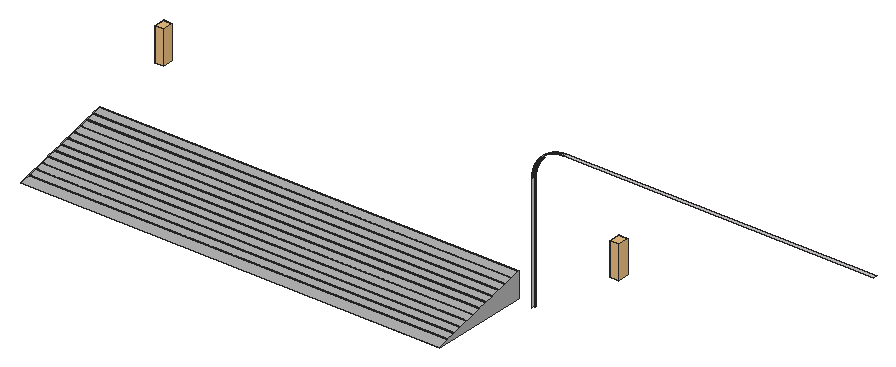
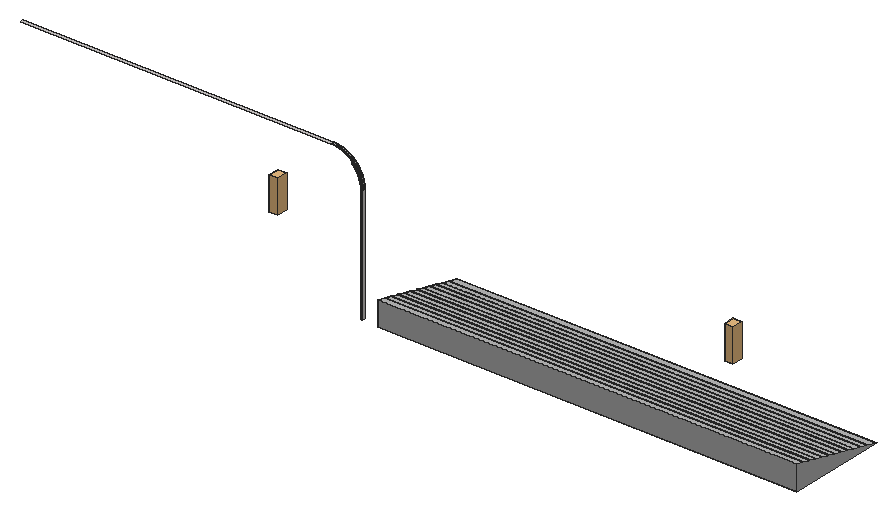
# SketchUp Ruby script. Lengths in inches.
U = 1.inch
M = Sketchup.active_model
def pt(a) = Geom::Point3d.new(a.map { |v| v * U })
def face(e, loops, mat)
  f = e.add_face(loops[0].map { |a| pt(a) })
  loops[1..].each { |l| e.add_face(l.map { |a| pt(a) }).erase! }
  f.material = f.back_material = mat if mat
  f
end
# faces: each face lists its corners as indices into pts; further lists are holes
def faces(e, pts, list, mat = nil) = list.each { |f| face(e, (f[0].is_a?(Array) ? f : [f]).map { |l| l.map { |i| pts[i] } }, mat) }
# xy, xz, yz: faces in a plane at the given z, y or x. An outline is a flat list of corners, or four numbers for a rectangle; further outlines are holes
def ring(l) = l.size == 4 ? [[l[0], l[1]], [l[2], l[1]], [l[2], l[3]], [l[0], l[3]]] : l.each_slice(2).to_a
def flat(e, list, mat, &to3) = list.each { |f| face(e, (f[0].is_a?(Array) ? f : [f]).map { |l| ring(l).map { |u, v| to3.(u, v) } }, mat) }
def xy(e, z, list, mat = nil) = flat(e, list, mat) { |x, y| [x, y, z] }
def xz(e, y, list, mat = nil) = flat(e, list, mat) { |x, z| [x, y, z] }
def yz(e, x, list, mat = nil) = flat(e, list, mat) { |y, z| [x, y, z] }
def lines(e, pts, list) = list.each { |a, b| e.add_line(pt(pts[a]), pt(pts[b])) }
# prism: a flat outline (further loops are holes) pulled along v
def prism(e, loops, v, mat = nil)
  f = face(e, loops, mat); d = Geom::Vector3d.new(v.map { |x| x * U })
  f.pushpull(f.normal.samedirection?(d) ? d.length : -d.length)
end
def box(e, o, s, mat = nil) = prism(e, [[o, [o[0] + s[0], o[1], o[2]], [o[0] + s[0], o[1] + s[1], o[2]], [o[0], o[1] + s[1], o[2]]]], [0, 0, s[2]], mat)
def at(x, y, z, deg = 0) = Geom::Transformation.translation(pt([x, y, z])) * Geom::Transformation.rotation(ORIGIN, Z_AXIS, deg.degrees)
def axes(o, x, y, z) = Geom::Transformation.new([*x, 0, *y, 0, *z, 0, *pt(o).to_a, 1])
def part(name) = M.definitions.add(name)
# library, detail: a bought-in or finely detailed component or shape, given as its bounding box
def library(name, o, s) = part(name).tap { |d| box(d.entities, o, s) }
def detail(e, o, s) = box(e.add_group.entities, o, s)
def put(e, d, t, mat = nil) = e.add_instance(d, t).tap { |i| i.material = mat if mat }
def group(e, t, mat = nil) = e.add_group.tap { |g| g.transformation = t; g.material = mat if mat }.entities
root = M.entities
M.materials.add("[Stone Vein Gray]").color = [206, 202, 201]
M.materials.add("[Terrazzo Tile Light]").color = [178, 178, 178]
c1 = library("WALL LIGHT 69",[4.19,4.05,-8.78],[4.61,5.7,17.13])
xy(root,0.35,[[172.85,83.25,173.15,83.5]])
xy(root,53.48,[[183.25,82.5,183.4,83.5]],"[Stone Vein Gray]")
xy(root,53.5,[[183.7,82.5,183.85,83.5],[183.85,82.5,184,83.5],[184,82.5,297,83.5]],"[Stone Vein Gray]")
xz(root,83.25,[[172.85,0,173.15,0.35]])
yz(root,172.5,[[82.5,0,83.5,42],[82.5,42,83.5,42.15],[82.5,42.15,83.5,42.3]],"[Stone Vein Gray]")
yz(root,172.52,[[82.5,42.6,83.5,42.75]],"[Stone Vein Gray]")
yz(root,172.85,[[83.25,0,83.5,0.35],[83.25,0.35,83.5,42],[83.25,42,83.5,42.15],[83.25,42.15,83.5,42.29]])
yz(root,173.15,[[83.25,0,83.5,0.35],[83.25,0.35,83.5,42],[83.25,42,83.5,42.14],[83.25,42.14,83.5,42.28]])
yz(root,173.16,[[83.25,42.43,83.5,42.57]])
p = [[172.51,83.5,42.45],[172.5,83.5,42.3],[172.5,82.5,42.3],[172.51,82.5,42.45],[172.85,83.5,42.29],[172.86,83.5,42.4375],
  [172.86,83.25,42.4375],[172.85,83.25,42.29],[173.16,83.5,42.43],[173.15,83.5,42.28],[173.15,83.25,42.28],[173.16,83.25,42.43],
  [172.87,83.5,42.58],[172.87,83.25,42.58],[172.52,83.5,42.6],[172.52,82.5,42.6],[172.875,83.5,42.73],[172.875,83.25,42.73],
  [173.17,83.5,42.71],[173.16,83.5,42.57],[173.16,83.25,42.57],[173.17,83.25,42.71],[172.88,83.5,42.875],[172.88,83.25,42.875],
  [173.18,83.5,42.85],[173.18,83.25,42.85],[172.54,83.5,42.9],[172.52,83.5,42.75],[172.52,82.5,42.75],[172.54,82.5,42.9],
  [172.55,83.5,43.05],[172.55,82.5,43.05],[172.9,83.5,43.02],[172.9,83.25,43.02],[173.2,83.5,42.99],[173.2,83.25,42.99],
  [172.91,83.5,43.17],[172.91,83.25,43.17],[173.21,83.5,43.13],[173.21,83.25,43.13],[172.5625,83.5,43.2],[172.5625,82.5,43.2],
  [173.23,83.5,43.28],[173.23,83.25,43.28],[172.58,83.5,43.35],[172.58,82.5,43.35],[172.93,83.5,43.3125],[172.93,83.25,43.3125],
  [172.95,83.5,43.46],[172.95,83.25,43.46],[173.24,83.5,43.42],[173.24,83.25,43.42],[172.6,83.5,43.5],[172.6,82.5,43.5],
  [173.26,83.5,43.56],[173.26,83.25,43.56],[172.62,83.5,43.65],[172.62,82.5,43.65],[172.97,83.5,43.6],[172.97,83.25,43.6],
  [172.99,83.5,43.74],[172.99,83.25,43.74],[173.28,83.5,43.7],[173.28,83.25,43.7],[172.64,83.5,43.8],[172.64,82.5,43.8],
  [173.01,83.5,43.89],[173.01,83.25,43.89],[173.31,83.5,43.84],[173.31,83.25,43.84],[172.67,83.5,43.95],[172.67,82.5,43.95],
  [173.33,83.5,43.98],[173.33,83.25,43.98],[172.69,83.5,44.1],[172.69,82.5,44.1],[173.04,83.5,44.03],[173.04,83.25,44.03],
  [173.0625,83.5,44.18],[173.0625,83.25,44.18],[173.36,83.5,44.12],[173.36,83.25,44.12],[172.72,83.5,44.24],[172.72,82.5,44.24],
  [173.39,83.5,44.26],[173.39,83.25,44.26],[172.75,83.5,44.39],[172.75,82.5,44.39],[173.09,83.5,44.32],[173.09,83.25,44.32],
  [173.125,83.5,44.46],[173.125,83.25,44.46],[173.42,83.5,44.39],[173.42,83.25,44.39],[172.78,83.5,44.54],[172.78,82.5,44.54],
  [173.45,83.5,44.53],[173.45,83.25,44.53],[172.82,83.5,44.68],[172.82,82.5,44.68],[173.16,83.5,44.6],[173.16,83.25,44.6],
  [173.48,83.5,44.67],[173.48,83.25,44.67],[173.19,83.5,44.74],[173.19,83.25,44.74],[172.85,83.5,44.83],[172.85,82.5,44.83],
  [173.23,83.5,44.89],[173.23,83.25,44.89],[173.52,83.5,44.81],[173.52,83.25,44.81],[172.89,83.5,44.98],[172.89,82.5,44.98],
  [173.56,83.5,44.95],[173.56,83.25,44.95],[173.27,83.5,45.03],[173.27,83.25,45.03],[173.6,83.5,45.08],[173.6,83.25,45.08],
  [172.93,83.5,45.12],[172.93,82.5,45.12],[173.31,83.5,45.17],[173.31,83.25,45.17],[172.97,83.5,45.27],[172.97,82.5,45.27],
  [173.64,83.5,45.22],[173.64,83.25,45.22],[173.35,83.5,45.31],[173.35,83.25,45.31],[173.68,83.5,45.35],[173.68,83.25,45.35],
  [173.02,83.5,45.41],[173.02,82.5,45.41],[173.4,83.5,45.45],[173.4,83.25,45.45],[173.0625,83.5,45.55],[173.0625,82.5,45.55],
  [173.44,83.5,45.58],[173.44,83.25,45.58],[173.73,83.5,45.49],[173.73,83.25,45.49],[173.77,83.5,45.62],[173.77,83.25,45.62],
  [173.11,83.5,45.7],[173.11,82.5,45.7],[173.49,83.5,45.72],[173.49,83.25,45.72],[173.82,83.5,45.76],[173.82,83.25,45.76],
  [173.16,83.5,45.84],[173.16,82.5,45.84],[173.54,83.5,45.86],[173.54,83.25,45.86],[173.21,83.5,45.98],[173.21,82.5,45.98],
  [173.87,83.5,45.89],[173.87,83.25,45.89],[173.59,83.5,46],[173.59,83.25,46],[173.92,83.5,46.02],[173.92,83.25,46.02],
  [173.26,83.5,46.12],[173.26,82.5,46.12],[173.64,83.5,46.13],[173.64,83.25,46.13],[173.98,83.5,46.15],[173.98,83.25,46.15],
  [173.32,83.5,46.26],[173.32,82.5,46.26],[173.7,83.5,46.27],[173.7,83.25,46.27],[174.03,83.5,46.28],[174.03,83.25,46.28],
  [173.375,83.5,46.4],[173.375,82.5,46.4],[173.76,83.5,46.4],[173.76,83.25,46.4],[174.09,83.5,46.41],[174.09,83.25,46.41],
  [173.43,83.5,46.54],[173.43,82.5,46.54],[173.8125,83.5,46.54],[173.8125,83.25,46.54],[174.15,83.5,46.54],[174.15,83.25,46.54],
  [173.49,83.5,46.68],[173.49,82.5,46.68],[173.875,83.5,46.67],[173.875,83.25,46.67],[174.21,83.5,46.67],[174.21,83.25,46.67],
  [173.56,83.5,46.81],[173.56,82.5,46.81],[173.9375,83.5,46.8],[173.9375,83.25,46.8],[174.27,83.5,46.8],[174.27,83.25,46.8],
  [173.62,83.5,46.95],[173.62,82.5,46.95],[174,83.5,46.93],[174,83.25,46.93],[174.33,83.5,46.93],[174.33,83.25,46.93],
  [174.07,83.5,47.0625],[174.07,83.25,47.0625],[174.4,83.5,47.05],[174.4,83.25,47.05],[173.6875,83.5,47.09],[173.6875,82.5,47.09],
  [173.75,83.5,47.22],[173.75,82.5,47.22],[174.13,83.5,47.19],[174.13,83.25,47.19],[174.46,83.5,47.18],[174.46,83.25,47.18],
  [173.82,83.5,47.35],[173.82,82.5,47.35],[174.2,83.5,47.32],[174.2,83.25,47.32],[174.53,83.5,47.3],[174.53,83.25,47.3],
  [174.27,83.5,47.45],[174.27,83.25,47.45],[174.6,83.5,47.42],[174.6,83.25,47.42],[173.89,83.5,47.49],[173.89,82.5,47.49],
  [174.34,83.5,47.57],[174.34,83.25,47.57],[174.68,83.5,47.55],[174.68,83.25,47.55],[173.97,83.5,47.62],[173.97,82.5,47.62],
  [174.75,83.5,47.67],[174.75,83.25,47.67],[174.04,83.5,47.75],[174.04,82.5,47.75],[174.42,83.5,47.7],[174.42,83.25,47.7],
  [174.49,83.5,47.83],[174.49,83.25,47.83],[174.82,83.5,47.79],[174.82,83.25,47.79],[174.12,83.5,47.88],[174.12,82.5,47.88],
  [174.57,83.5,47.95],[174.57,83.25,47.95],[174.9,83.5,47.91],[174.9,83.25,47.91],[174.19,83.5,48.01],[174.19,82.5,48.01],
  [174.65,83.5,48.07],[174.65,83.25,48.07],[174.98,83.5,48.03],[174.98,83.25,48.03],[174.27,83.5,48.14],[174.27,82.5,48.14],
  [175.06,83.5,48.15],[175.06,83.25,48.15],[174.36,83.5,48.26],[174.36,82.5,48.26],[174.73,83.5,48.19],[174.73,83.25,48.19],
  [175.14,83.5,48.26],[175.14,83.25,48.26],[174.8125,83.5,48.32],[174.8125,83.25,48.32],[174.4375,83.5,48.39],[174.4375,82.5,48.39],
  [174.89,83.5,48.44],[174.89,83.25,48.44],[175.22,83.5,48.38],[175.22,83.25,48.38],[174.52,83.5,48.51],[174.52,82.5,48.51],
  [174.98,83.5,48.55],[174.98,83.25,48.55],[175.31,83.5,48.49],[175.31,83.25,48.49],[174.61,83.5,48.64],[174.61,82.5,48.64],
  [175.39,83.5,48.61],[175.39,83.25,48.61],[174.7,83.5,48.76],[174.7,82.5,48.76],[175.07,83.5,48.67],[175.07,83.25,48.67],
  [175.48,83.5,48.72],[175.48,83.25,48.72],[175.15,83.5,48.79],[175.15,83.25,48.79],[175.57,83.5,48.83],[175.57,83.25,48.83],
  [174.79,83.5,48.88],[174.79,82.5,48.88],[175.24,83.5,48.9],[175.24,83.25,48.9],[175.66,83.5,48.9375],[175.66,83.25,48.9375],
  [174.875,83.5,49],[174.875,82.5,49],[175.33,83.5,49.02],[175.33,83.25,49.02],[175.75,83.5,49.05],[175.75,83.25,49.05],
  [174.97,83.5,49.12],[174.97,82.5,49.12],[175.43,83.5,49.13],[175.43,83.25,49.13],[175.84,83.5,49.15],[175.84,83.25,49.15],
  [175.0625,83.5,49.24],[175.0625,82.5,49.24],[175.52,83.5,49.24],[175.52,83.25,49.24],[175.16,83.5,49.35],[175.16,82.5,49.35],
  [175.62,83.5,49.35],[175.62,83.25,49.35],[175.9375,83.5,49.26],[175.9375,83.25,49.26],[176.03,83.5,49.36],[176.03,83.25,49.36],
  [175.26,83.5,49.47],[175.26,82.5,49.47],[175.71,83.5,49.46],[175.71,83.25,49.46],[176.13,83.5,49.47],[176.13,83.25,49.47],
  [175.35,83.5,49.58],[175.35,82.5,49.58],[175.8125,83.5,49.57],[175.8125,83.25,49.57],[176.23,83.5,49.57],[176.23,83.25,49.57],
  [175.45,83.5,49.7],[175.45,82.5,49.7],[175.91,83.5,49.68],[175.91,83.25,49.68],[176.33,83.5,49.67],[176.33,83.25,49.67],
  [175.56,83.5,49.81],[175.56,82.5,49.81],[176.01,83.5,49.78],[176.01,83.25,49.78],[176.43,83.5,49.77],[176.43,83.25,49.77],
  [175.66,83.5,49.92],[175.66,82.5,49.92],[176.53,83.5,49.87],[176.53,83.25,49.87],[175.76,83.5,50.02],[175.76,82.5,50.02],
  [175.87,83.5,50.13],[175.87,82.5,50.13],[175.98,83.5,50.24],[175.98,82.5,50.24],[176.08,83.5,50.34],[176.08,82.5,50.34],
  [176.19,83.5,50.44],[176.19,82.5,50.44],[176.3,83.5,50.55],[176.3,82.5,50.55],[176.42,83.5,50.65],[176.42,82.5,50.65],
  [176.53,83.5,50.74],[176.53,82.5,50.74],[176.65,83.5,50.84],[176.65,82.5,50.84],[176.76,83.5,50.9375],[176.76,82.5,50.9375],
  [176.88,83.5,51.03],[176.88,82.5,51.03],[177,83.5,51.125],[177,82.5,51.125],[177.12,83.5,51.21],[177.12,82.5,51.21],
  [177.24,83.5,51.3],[177.24,82.5,51.3],[177.36,83.5,51.39],[177.36,82.5,51.39],[177.49,83.5,51.48],[177.49,82.5,51.48],
  [177.61,83.5,51.5625],[177.61,82.5,51.5625],[177.74,83.5,51.64],[177.74,82.5,51.64],[177.86,83.5,51.73],[177.86,82.5,51.73],
  [177.99,83.5,51.81],[177.99,82.5,51.81],[178.12,83.5,51.88],[178.12,82.5,51.88],[178.25,83.5,51.96],[178.25,82.5,51.96],
  [178.38,83.5,52.03],[178.38,82.5,52.03],[178.51,83.5,52.11],[178.51,82.5,52.11],[178.65,83.5,52.18],[178.65,82.5,52.18],
  [178.78,83.5,52.25],[178.78,82.5,52.25],[178.91,83.5,52.3125],[178.91,82.5,52.3125],[179.05,83.5,52.38],[179.05,82.5,52.38],
  [179.19,83.5,52.44],[179.19,82.5,52.44],[179.32,83.5,52.51],[179.32,82.5,52.51],[179.46,83.5,52.57],[179.46,82.5,52.57],
  [179.6,83.5,52.625],[179.6,82.5,52.625],[179.74,83.5,52.68],[179.74,82.5,52.68],[179.88,83.5,52.74],[179.88,82.5,52.74],
  [180.02,83.5,52.79],[180.02,82.5,52.79],[180.16,83.5,52.84],[180.16,82.5,52.84],[180.3,83.5,52.89],[180.3,82.5,52.89],
  [180.45,83.5,52.9375],[180.45,82.5,52.9375],[180.59,83.5,52.98],[180.59,82.5,52.98],[180.73,83.5,53.03],[180.73,82.5,53.03],
  [180.88,83.5,53.07],[180.88,82.5,53.07],[181.02,83.5,53.11],[181.02,82.5,53.11],[181.17,83.5,53.15],[181.17,82.5,53.15],
  [181.32,83.5,53.18],[181.32,82.5,53.18],[181.46,83.5,53.22],[181.46,82.5,53.22],[181.61,83.5,53.25],[181.61,82.5,53.25],
  [181.76,83.5,53.28],[181.76,82.5,53.28],[181.9,83.5,53.31],[181.9,82.5,53.31],[182.05,83.5,53.33],[182.05,82.5,53.33],
  [182.2,83.5,53.36],[182.2,82.5,53.36],[182.35,83.5,53.38],[182.35,82.5,53.38],[182.5,83.5,53.4],[182.5,82.5,53.4],
  [182.65,83.5,53.42],[182.65,82.5,53.42],[182.8,83.5,53.4375],[182.8,82.5,53.4375],[182.95,83.5,53.45],[182.95,82.5,53.45],
  [183.1,83.5,53.46],[183.1,82.5,53.46],[183.25,83.5,53.48],[183.25,82.5,53.48],[183.55,83.5,53.49],[183.4,83.5,53.48],
  [183.4,82.5,53.48],[183.55,82.5,53.49],[183.7,83.5,53.5],[183.7,82.5,53.5]]
faces(root,p,[[0,1,2,3],[14,0,3,15],[26,27,28,29],[30,26,29,31],[40,30,31,41],[44,40,41,45],[52,44,45,53],[56,52,53,57],
  [64,56,57,65],[70,64,65,71],[74,70,71,75],[82,74,75,83],[86,82,83,87],[94,86,87,95],[98,94,95,99],[106,98,99,107],
  [112,106,107,113],[120,112,113,121],[124,120,121,125],[132,124,125,133],[136,132,133,137],[144,136,137,145],[150,144,145,151],[154,150,151,155],
  [162,154,155,163],[168,162,163,169],[174,168,169,175],[180,174,175,181],[186,180,181,187],[192,186,187,193],[198,192,193,199],[208,198,199,209],
  [210,208,209,211],[216,210,211,217],[226,216,217,227],[232,226,227,233],[236,232,233,237],[244,236,237,245],[250,244,245,251],[256,250,251,257],
  [260,256,257,261],[268,260,261,269],[274,268,269,275],[280,274,275,281],[284,280,281,285],[294,284,285,295],[300,294,295,301],[306,300,301,307],
  [312,306,307,313],[316,312,313,317],[324,316,317,325],[330,324,325,331],[336,330,331,337],[342,336,337,343],[348,342,343,349],[352,348,349,353],
  [354,352,353,355],[356,354,355,357],[358,356,357,359],[360,358,359,361],[362,360,361,363],[364,362,363,365],[366,364,365,367],[368,366,367,369],
  [370,368,369,371],[372,370,371,373],[374,372,373,375],[376,374,375,377],[378,376,377,379],[380,378,379,381],[382,380,381,383],[384,382,383,385],
  [386,384,385,387],[388,386,387,389],[390,388,389,391],[392,390,391,393],[394,392,393,395],[396,394,395,397],[398,396,397,399],[400,398,399,401],
  [402,400,401,403],[404,402,403,405],[406,404,405,407],[408,406,407,409],[410,408,409,411],[412,410,411,413],[414,412,413,415],[416,414,415,417],
  [418,416,417,419],[420,418,419,421],[422,420,421,423],[424,422,423,425],[426,424,425,427],[428,426,427,429],[430,428,429,431],[432,430,431,433],
  [434,432,433,435],[436,434,435,437],[438,436,437,439],[440,438,439,441],[442,440,441,443],[444,442,443,445],[446,444,445,447],[448,446,447,449],
  [450,448,449,451],[452,450,451,453],[454,452,453,455],[456,454,455,457],[458,456,457,459],[460,458,459,461],[462,460,461,463],[464,462,463,465],
  [466,467,468,469],[470,466,469,471]],"[Stone Vein Gray]")
faces(root,p,[[4,5,6,7],[8,9,10,11],[5,12,13,6],[12,16,17,13],[18,19,20,21],[16,22,23,17],[24,18,21,25],[22,32,33,23],
  [34,24,25,35],[32,36,37,33],[38,34,35,39],[42,38,39,43],[36,46,47,37],[46,48,49,47],[50,42,43,51],[54,50,51,55],
  [48,58,59,49],[58,60,61,59],[62,54,55,63],[60,66,67,61],[68,62,63,69],[72,68,69,73],[66,76,77,67],[76,78,79,77],
  [80,72,73,81],[84,80,81,85],[78,88,89,79],[88,90,91,89],[92,84,85,93],[96,92,93,97],[90,100,101,91],[102,96,97,103],
  [100,104,105,101],[104,108,109,105],[110,102,103,111],[114,110,111,115],[108,116,117,109],[118,114,115,119],[116,122,123,117],[126,118,119,127],
  [122,128,129,123],[130,126,127,131],[128,134,135,129],[134,138,139,135],[140,130,131,141],[142,140,141,143],[138,146,147,139],[148,142,143,149],
  [146,152,153,147],[156,148,149,157],[152,158,159,153],[160,156,157,161],[158,164,165,159],[166,160,161,167],[164,170,171,165],[172,166,167,173],
  [170,176,177,171],[178,172,173,179],[176,182,183,177],[184,178,179,185],[182,188,189,183],[190,184,185,191],[188,194,195,189],[196,190,191,197],
  [194,200,201,195],[202,196,197,203],[200,204,205,201],[206,202,203,207],[204,212,213,205],[214,206,207,215],[212,218,219,213],[220,214,215,221],
  [218,222,223,219],[224,220,221,225],[222,228,229,223],[230,224,225,231],[234,230,231,235],[228,238,239,229],[238,240,241,239],[242,234,235,243],
  [240,246,247,241],[248,242,243,249],[246,252,253,247],[254,248,249,255],[258,254,255,259],[252,262,263,253],[264,258,259,265],[262,266,267,263],
  [266,270,271,267],[272,264,265,273],[270,276,277,271],[278,272,273,279],[282,278,279,283],[276,286,287,277],[288,282,283,289],[286,290,291,287],
  [292,288,289,293],[290,296,297,291],[298,292,293,299],[296,302,303,297],[304,298,299,305],[302,308,309,303],[310,304,305,311],[308,314,315,309],
  [314,318,319,315],[320,310,311,321],[322,320,321,323],[318,326,327,319],[328,322,323,329],[326,332,333,327],[334,328,329,335],[332,338,339,333],
  [340,334,335,341],[338,344,345,339],[346,340,341,347],[350,346,347,351]])
put(root,c1,axes([34.29,77.18,39.58],[0.7,0,0],[0,0.7,0],[0,0,0.7]))
g1 = group(root,at(62,84,0),"[Terrazzo Tile Light]")
prism(g1,[[[-48,-5.82,7.54],[-48,-3.16,8.21],[-48,-3.16,8.12],[-48,-2.91,8.12],[-48,-2.91,8.27],[-48,0,9],[-48,0,0],[-48,-36,0],[-48,-32.26,0.93],[-48,-32.26,0.85],[-48,-32.01,0.85],[-48,-32.01,1],[-48,-29.35,1.66],[-48,-29.35,1.57],[-48,-29.1,1.57],[-48,-29.1,1.72],[-48,-26.44,2.39],[-48,-26.44,2.3],[-48,-26.19,2.3],[-48,-26.19,2.45],[-48,-23.53,3.12],[-48,-23.53,3.03],[-48,-23.28,3.03],[-48,-23.28,3.18],[-48,-20.62,3.84],[-48,-20.62,3.76],[-48,-20.37,3.76],[-48,-20.37,3.91],[-48,-17.71,4.57],[-48,-17.71,4.48],[-48,-17.46,4.48],[-48,-17.46,4.63],[-48,-14.8,5.3],[-48,-14.8,5.21],[-48,-14.55,5.21],[-48,-14.55,5.36],[-48,-11.89,6.03],[-48,-11.89,5.94],[-48,-11.64,5.94],[-48,-11.64,6.09],[-48,-8.98,6.75],[-48,-8.98,6.67],[-48,-8.73,6.67],[-48,-8.73,6.82],[-48,-6.07,7.48],[-48,-6.07,7.39],[-48,-5.82,7.39]]],[152.5,0,0])
put(root,c1,axes([201.07,75.68,28.83],[0.7,0,0],[0,0.7,0],[0,0,0.7]))
